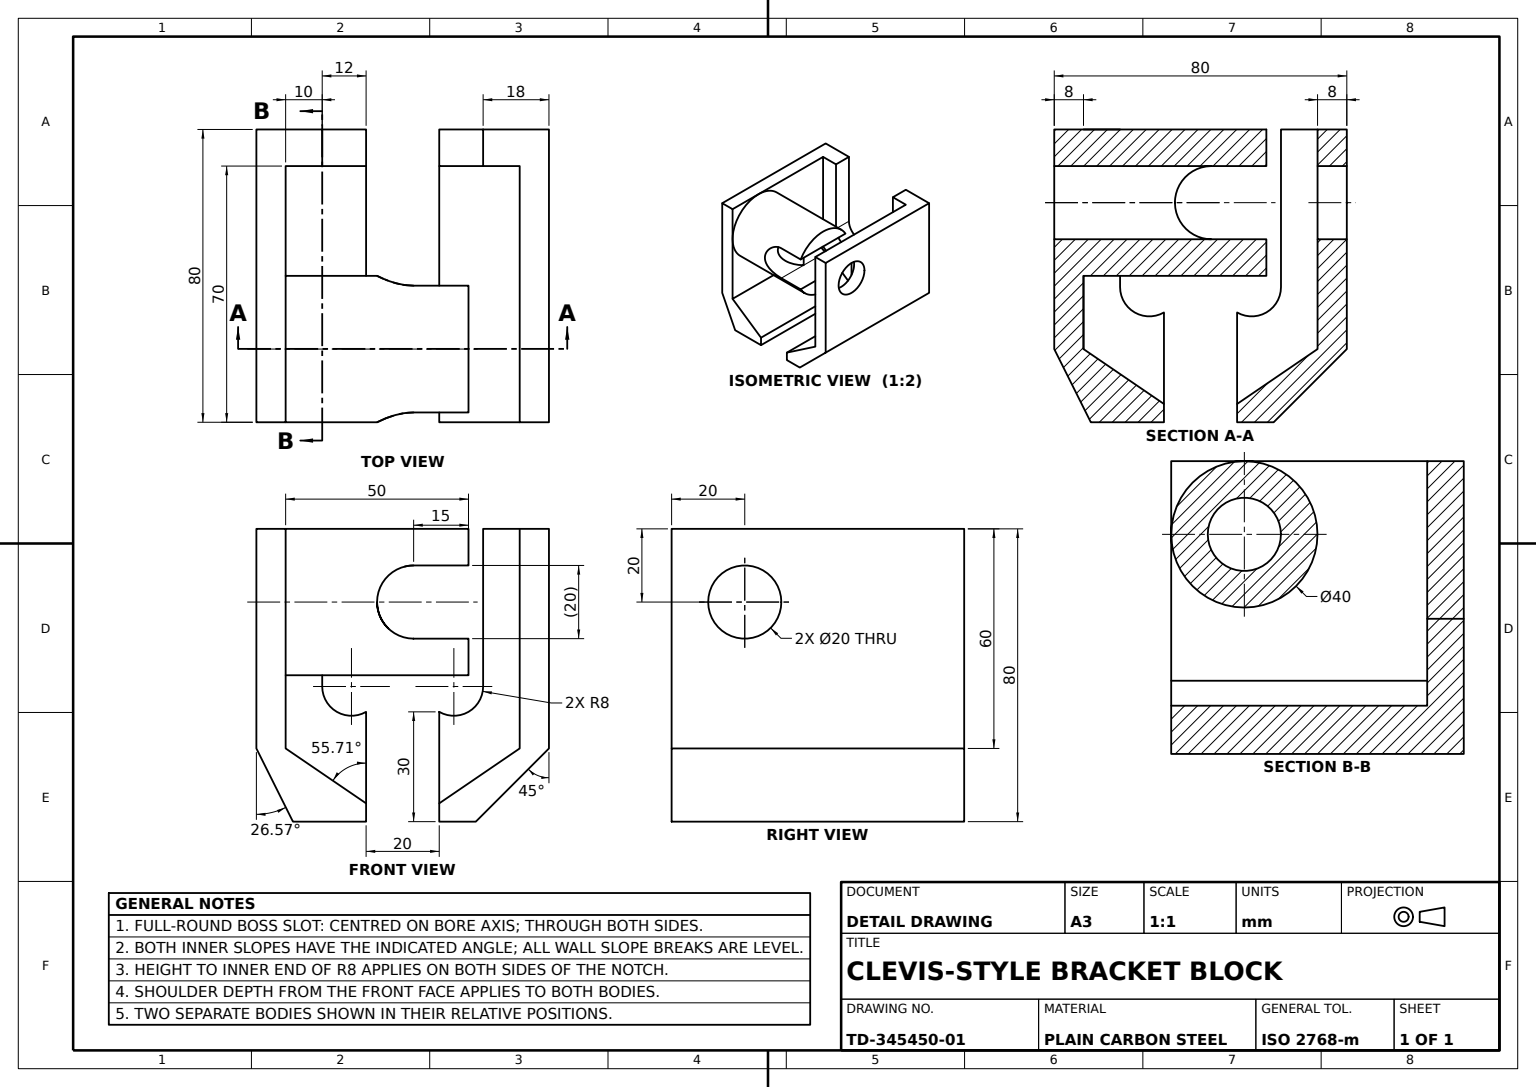
ISO-10303-21;
HEADER;
FILE_DESCRIPTION((''),'2;1');
FILE_NAME('','',(''),(''),'','','');
FILE_SCHEMA(('AUTOMOTIVE_DESIGN'));
ENDSEC;
DATA;
#1=APPLICATION_CONTEXT('');
#2=PRODUCT_CONTEXT('',#1,'mechanical');
#3=PRODUCT('','','',(#2));
#4=PRODUCT_DEFINITION_FORMATION('','',#3);
#5=PRODUCT_DEFINITION_CONTEXT('',#1,'design');
#6=PRODUCT_DEFINITION('','',#4,#5);
#7=PRODUCT_DEFINITION_SHAPE('','',#6);
#8=(LENGTH_UNIT()NAMED_UNIT(*)SI_UNIT(.MILLI.,.METRE.));
#9=(NAMED_UNIT(*)PLANE_ANGLE_UNIT()SI_UNIT($,.RADIAN.));
#10=(NAMED_UNIT(*)SI_UNIT($,.STERADIAN.)SOLID_ANGLE_UNIT());
#11=UNCERTAINTY_MEASURE_WITH_UNIT(LENGTH_MEASURE(1.E-05),#8,'distance_accuracy_value','');
#12=(GEOMETRIC_REPRESENTATION_CONTEXT(3)GLOBAL_UNCERTAINTY_ASSIGNED_CONTEXT((#11))GLOBAL_UNIT_ASSIGNED_CONTEXT((#8,#9,#10))REPRESENTATION_CONTEXT('',''));
#13=CARTESIAN_POINT('',(-40.,20.,42.));
#14=VERTEX_POINT('',#13);
#15=CARTESIAN_POINT('',(-40.,80.,42.));
#16=VERTEX_POINT('',#15);
#17=DIRECTION('',(0.,1.,0.));
#18=VECTOR('',#17,1000.);
#19=LINE('',#13,#18);
#20=EDGE_CURVE('',#14,#16,#19,.T.);
#21=ORIENTED_EDGE('',*,*,#20,.F.);
#22=CARTESIAN_POINT('',(-40.,5.,20.));
#23=VERTEX_POINT('',#22);
#24=DIRECTION('',(0.,0.563336825,0.826227343));
#25=VECTOR('',#24,1000.);
#26=LINE('',#22,#25);
#27=EDGE_CURVE('',#23,#14,#26,.T.);
#28=ORIENTED_EDGE('',*,*,#27,.F.);
#29=CARTESIAN_POINT('',(-40.,0.,20.));
#30=VERTEX_POINT('',#29);
#31=LINE('',#29,#18);
#32=EDGE_CURVE('',#30,#23,#31,.T.);
#33=ORIENTED_EDGE('',*,*,#32,.F.);
#34=CARTESIAN_POINT('',(-40.,0.,30.));
#35=VERTEX_POINT('',#34);
#36=CARTESIAN_POINT('',(-40.,0.,0.));
#37=DIRECTION('',(0.,0.,1.));
#38=VECTOR('',#37,1000.);
#39=LINE('',#36,#38);
#40=EDGE_CURVE('',#30,#35,#39,.T.);
#41=ORIENTED_EDGE('',*,*,#40,.T.);
#42=CARTESIAN_POINT('',(-40.,20.,50.));
#43=VERTEX_POINT('',#42);
#44=CARTESIAN_POINT('',(-40.,-15.,15.));
#45=DIRECTION('',(0.,-0.707106781,-0.707106781));
#46=VECTOR('',#45,1000.);
#47=LINE('',#44,#46);
#48=EDGE_CURVE('',#43,#35,#47,.T.);
#49=ORIENTED_EDGE('',*,*,#48,.F.);
#50=CARTESIAN_POINT('',(-40.,80.,50.));
#51=VERTEX_POINT('',#50);
#52=CARTESIAN_POINT('',(-40.,0.,50.));
#53=LINE('',#52,#18);
#54=EDGE_CURVE('',#43,#51,#53,.T.);
#55=ORIENTED_EDGE('',*,*,#54,.T.);
#56=CARTESIAN_POINT('',(-40.,80.,0.));
#57=DIRECTION('',(0.,0.,-1.));
#58=VECTOR('',#57,1000.);
#59=LINE('',#56,#58);
#60=EDGE_CURVE('',#51,#16,#59,.T.);
#61=ORIENTED_EDGE('',*,*,#60,.T.);
#62=EDGE_LOOP('',(#21,#28,#33,#41,#49,#55,#61));
#63=FACE_OUTER_BOUND('',#62,.T.);
#64=DIRECTION('',(1.,0.,0.));
#65=AXIS2_PLACEMENT_3D('',#36,#64,#57);
#66=PLANE('',#65);
#67=ADVANCED_FACE('',(#63),#66,.F.);
#68=CARTESIAN_POINT('',(-10.,60.,50.));
#69=VERTEX_POINT('',#68);
#70=CARTESIAN_POINT('',(-30.,60.,50.));
#71=VERTEX_POINT('',#70);
#72=CARTESIAN_POINT('',(-20.,60.,50.));
#73=DIRECTION('',(-1.,0.,0.));
#74=AXIS2_PLACEMENT_3D('',#72,#57,#73);
#75=CIRCLE('',#74,10.);
#76=EDGE_CURVE('',#69,#71,#75,.T.);
#77=ORIENTED_EDGE('',*,*,#76,.F.);
#78=CARTESIAN_POINT('',(-10.,60.,42.));
#79=VERTEX_POINT('',#78);
#80=CARTESIAN_POINT('',(-10.,60.,58.));
#81=LINE('',#80,#58);
#82=EDGE_CURVE('',#69,#79,#81,.T.);
#83=ORIENTED_EDGE('',*,*,#82,.T.);
#84=CARTESIAN_POINT('',(-30.,60.,42.));
#85=VERTEX_POINT('',#84);
#86=CARTESIAN_POINT('',(-20.,60.,42.));
#87=AXIS2_PLACEMENT_3D('',#86,#37,#64);
#88=CIRCLE('',#87,10.);
#89=EDGE_CURVE('',#85,#79,#88,.T.);
#90=ORIENTED_EDGE('',*,*,#89,.F.);
#91=CARTESIAN_POINT('',(-30.,60.,58.));
#92=LINE('',#91,#58);
#93=EDGE_CURVE('',#71,#85,#92,.T.);
#94=ORIENTED_EDGE('',*,*,#93,.F.);
#95=EDGE_LOOP('',(#77,#83,#90,#94));
#96=FACE_OUTER_BOUND('',#95,.T.);
#97=CARTESIAN_POINT('',(-20.,60.,58.));
#98=AXIS2_PLACEMENT_3D('',#97,#57,#73);
#99=CYLINDRICAL_SURFACE('',#98,10.);
#100=ADVANCED_FACE('',(#96),#99,.F.);
#101=CARTESIAN_POINT('',(30.,80.,42.));
#102=VERTEX_POINT('',#101);
#103=CARTESIAN_POINT('',(30.,80.,32.));
#104=VERTEX_POINT('',#103);
#105=CARTESIAN_POINT('',(30.,80.,12.853653));
#106=LINE('',#105,#58);
#107=EDGE_CURVE('',#102,#104,#106,.T.);
#108=ORIENTED_EDGE('',*,*,#107,.T.);
#109=CARTESIAN_POINT('',(30.,36.928203,32.));
#110=VERTEX_POINT('',#109);
#111=CARTESIAN_POINT('',(30.,0.,32.));
#112=LINE('',#111,#18);
#113=EDGE_CURVE('',#110,#104,#112,.T.);
#114=ORIENTED_EDGE('',*,*,#113,.F.);
#115=CARTESIAN_POINT('',(30.,30.,20.));
#116=VERTEX_POINT('',#115);
#117=CARTESIAN_POINT('',(30.,36.928203,24.));
#118=AXIS2_PLACEMENT_3D('',#117,#73,#57);
#119=CIRCLE('',#118,8.);
#120=EDGE_CURVE('',#116,#110,#119,.T.);
#121=ORIENTED_EDGE('',*,*,#120,.F.);
#122=CARTESIAN_POINT('',(30.,5.,20.));
#123=VERTEX_POINT('',#122);
#124=CARTESIAN_POINT('',(30.,0.,20.));
#125=DIRECTION('',(0.,-1.,0.));
#126=VECTOR('',#125,1000.);
#127=LINE('',#124,#126);
#128=EDGE_CURVE('',#116,#123,#127,.T.);
#129=ORIENTED_EDGE('',*,*,#128,.T.);
#130=CARTESIAN_POINT('',(30.,20.,42.));
#131=VERTEX_POINT('',#130);
#132=LINE('',#122,#25);
#133=EDGE_CURVE('',#123,#131,#132,.T.);
#134=ORIENTED_EDGE('',*,*,#133,.T.);
#135=LINE('',#130,#18);
#136=EDGE_CURVE('',#131,#102,#135,.T.);
#137=ORIENTED_EDGE('',*,*,#136,.T.);
#138=EDGE_LOOP('',(#108,#114,#121,#129,#134,#137));
#139=FACE_OUTER_BOUND('',#138,.T.);
#140=CARTESIAN_POINT('',(30.,20.,12.853653));
#141=AXIS2_PLACEMENT_3D('',#140,#64,#57);
#142=PLANE('',#141);
#143=ADVANCED_FACE('',(#139),#142,.F.);
#144=ORIENTED_EDGE('',*,*,#82,.F.);
#145=EDGE_CURVE('',#71,#69,#75,.T.);
#146=ORIENTED_EDGE('',*,*,#145,.F.);
#147=ORIENTED_EDGE('',*,*,#93,.T.);
#148=EDGE_CURVE('',#79,#85,#88,.T.);
#149=ORIENTED_EDGE('',*,*,#148,.F.);
#150=EDGE_LOOP('',(#144,#146,#147,#149));
#151=FACE_OUTER_BOUND('',#150,.T.);
#152=ADVANCED_FACE('',(#151),#99,.F.);
#153=ORIENTED_EDGE('',*,*,#89,.T.);
#154=ORIENTED_EDGE('',*,*,#148,.T.);
#155=EDGE_LOOP('',(#153,#154));
#156=FACE_BOUND('',#155,.T.);
#157=VECTOR('',#64,1000.);
#158=LINE('',#13,#157);
#159=EDGE_CURVE('',#14,#131,#158,.T.);
#160=ORIENTED_EDGE('',*,*,#159,.F.);
#161=ORIENTED_EDGE('',*,*,#20,.T.);
#162=LINE('',#15,#157);
#163=EDGE_CURVE('',#16,#102,#162,.T.);
#164=ORIENTED_EDGE('',*,*,#163,.T.);
#165=ORIENTED_EDGE('',*,*,#136,.F.);
#166=EDGE_LOOP('',(#160,#161,#164,#165));
#167=FACE_OUTER_BOUND('',#166,.T.);
#168=AXIS2_PLACEMENT_3D('',#13,#37,#64);
#169=PLANE('',#168);
#170=ADVANCED_FACE('',(#156,#167),#169,.F.);
#171=CARTESIAN_POINT('',(40.,0.,30.));
#172=VERTEX_POINT('',#171);
#173=LINE('',#34,#157);
#174=EDGE_CURVE('',#35,#172,#173,.T.);
#175=ORIENTED_EDGE('',*,*,#174,.F.);
#176=ORIENTED_EDGE('',*,*,#40,.F.);
#177=CARTESIAN_POINT('',(40.,0.,20.));
#178=VERTEX_POINT('',#177);
#179=LINE('',#29,#157);
#180=EDGE_CURVE('',#30,#178,#179,.T.);
#181=ORIENTED_EDGE('',*,*,#180,.T.);
#182=CARTESIAN_POINT('',(40.,0.,0.));
#183=LINE('',#182,#38);
#184=EDGE_CURVE('',#178,#172,#183,.T.);
#185=ORIENTED_EDGE('',*,*,#184,.T.);
#186=EDGE_LOOP('',(#175,#176,#181,#185));
#187=FACE_OUTER_BOUND('',#186,.T.);
#188=AXIS2_PLACEMENT_3D('',#36,#17,#37);
#189=PLANE('',#188);
#190=ADVANCED_FACE('',(#187),#189,.F.);
#191=ORIENTED_EDGE('',*,*,#76,.T.);
#192=ORIENTED_EDGE('',*,*,#145,.T.);
#193=EDGE_LOOP('',(#191,#192));
#194=FACE_BOUND('',#193,.T.);
#195=CARTESIAN_POINT('',(40.,80.,50.));
#196=VERTEX_POINT('',#195);
#197=LINE('',#50,#157);
#198=EDGE_CURVE('',#51,#196,#197,.T.);
#199=ORIENTED_EDGE('',*,*,#198,.F.);
#200=ORIENTED_EDGE('',*,*,#54,.F.);
#201=CARTESIAN_POINT('',(40.,20.,50.));
#202=VERTEX_POINT('',#201);
#203=LINE('',#42,#157);
#204=EDGE_CURVE('',#43,#202,#203,.T.);
#205=ORIENTED_EDGE('',*,*,#204,.T.);
#206=CARTESIAN_POINT('',(40.,0.,50.));
#207=LINE('',#206,#18);
#208=EDGE_CURVE('',#202,#196,#207,.T.);
#209=ORIENTED_EDGE('',*,*,#208,.T.);
#210=EDGE_LOOP('',(#199,#200,#205,#209));
#211=FACE_OUTER_BOUND('',#210,.T.);
#212=AXIS2_PLACEMENT_3D('',#52,#57,#73);
#213=PLANE('',#212);
#214=ADVANCED_FACE('',(#194,#211),#213,.F.);
#215=ORIENTED_EDGE('',*,*,#32,.T.);
#216=VECTOR('',#73,1000.);
#217=LINE('',#122,#216);
#218=EDGE_CURVE('',#123,#23,#217,.T.);
#219=ORIENTED_EDGE('',*,*,#218,.F.);
#220=ORIENTED_EDGE('',*,*,#128,.F.);
#221=CARTESIAN_POINT('',(40.,30.,20.));
#222=VERTEX_POINT('',#221);
#223=CARTESIAN_POINT('',(-40.,30.,20.));
#224=LINE('',#223,#157);
#225=EDGE_CURVE('',#116,#222,#224,.T.);
#226=ORIENTED_EDGE('',*,*,#225,.T.);
#227=LINE('',#177,#18);
#228=EDGE_CURVE('',#178,#222,#227,.T.);
#229=ORIENTED_EDGE('',*,*,#228,.F.);
#230=ORIENTED_EDGE('',*,*,#180,.F.);
#231=EDGE_LOOP('',(#215,#219,#220,#226,#229,#230));
#232=FACE_OUTER_BOUND('',#231,.T.);
#233=AXIS2_PLACEMENT_3D('',#29,#57,#73);
#234=PLANE('',#233);
#235=ADVANCED_FACE('',(#232),#234,.T.);
#236=ORIENTED_EDGE('',*,*,#133,.F.);
#237=ORIENTED_EDGE('',*,*,#218,.T.);
#238=ORIENTED_EDGE('',*,*,#27,.T.);
#239=ORIENTED_EDGE('',*,*,#159,.T.);
#240=EDGE_LOOP('',(#236,#237,#238,#239));
#241=FACE_OUTER_BOUND('',#240,.T.);
#242=DIRECTION('',(0.,-0.826227343,0.563336825));
#243=DIRECTION('',(0.,-0.563336825,-0.826227343));
#244=AXIS2_PLACEMENT_3D('',#122,#242,#243);
#245=PLANE('',#244);
#246=ADVANCED_FACE('',(#241),#245,.F.);
#247=ORIENTED_EDGE('',*,*,#60,.F.);
#248=ORIENTED_EDGE('',*,*,#198,.T.);
#249=CARTESIAN_POINT('',(40.,80.,32.));
#250=VERTEX_POINT('',#249);
#251=CARTESIAN_POINT('',(40.,80.,0.));
#252=LINE('',#251,#58);
#253=EDGE_CURVE('',#196,#250,#252,.T.);
#254=ORIENTED_EDGE('',*,*,#253,.T.);
#255=CARTESIAN_POINT('',(-40.,80.,32.));
#256=LINE('',#255,#157);
#257=EDGE_CURVE('',#104,#250,#256,.T.);
#258=ORIENTED_EDGE('',*,*,#257,.F.);
#259=ORIENTED_EDGE('',*,*,#107,.F.);
#260=ORIENTED_EDGE('',*,*,#163,.F.);
#261=EDGE_LOOP('',(#247,#248,#254,#258,#259,#260));
#262=FACE_OUTER_BOUND('',#261,.T.);
#263=AXIS2_PLACEMENT_3D('',#56,#125,#57);
#264=PLANE('',#263);
#265=ADVANCED_FACE('',(#262),#264,.F.);
#266=ORIENTED_EDGE('',*,*,#204,.F.);
#267=ORIENTED_EDGE('',*,*,#48,.T.);
#268=ORIENTED_EDGE('',*,*,#174,.T.);
#269=CARTESIAN_POINT('',(40.,-15.,15.));
#270=LINE('',#269,#46);
#271=EDGE_CURVE('',#202,#172,#270,.T.);
#272=ORIENTED_EDGE('',*,*,#271,.F.);
#273=EDGE_LOOP('',(#266,#267,#268,#272));
#274=FACE_OUTER_BOUND('',#273,.T.);
#275=DIRECTION('',(0.,-0.707106781,0.707106781));
#276=AXIS2_PLACEMENT_3D('',#44,#275,#45);
#277=PLANE('',#276);
#278=ADVANCED_FACE('',(#274),#277,.T.);
#279=ORIENTED_EDGE('',*,*,#228,.T.);
#280=CARTESIAN_POINT('',(40.,36.928203,32.));
#281=VERTEX_POINT('',#280);
#282=CARTESIAN_POINT('',(40.,36.928203,24.));
#283=AXIS2_PLACEMENT_3D('',#282,#64,#57);
#284=CIRCLE('',#283,8.);
#285=EDGE_CURVE('',#281,#222,#284,.T.);
#286=ORIENTED_EDGE('',*,*,#285,.F.);
#287=CARTESIAN_POINT('',(40.,0.,32.));
#288=LINE('',#287,#126);
#289=EDGE_CURVE('',#250,#281,#288,.T.);
#290=ORIENTED_EDGE('',*,*,#289,.F.);
#291=ORIENTED_EDGE('',*,*,#253,.F.);
#292=ORIENTED_EDGE('',*,*,#208,.F.);
#293=ORIENTED_EDGE('',*,*,#271,.T.);
#294=ORIENTED_EDGE('',*,*,#184,.F.);
#295=EDGE_LOOP('',(#279,#286,#290,#291,#292,#293,#294));
#296=FACE_OUTER_BOUND('',#295,.T.);
#297=AXIS2_PLACEMENT_3D('',#182,#64,#57);
#298=PLANE('',#297);
#299=ADVANCED_FACE('',(#296),#298,.T.);
#300=ORIENTED_EDGE('',*,*,#113,.T.);
#301=ORIENTED_EDGE('',*,*,#257,.T.);
#302=ORIENTED_EDGE('',*,*,#289,.T.);
#303=CARTESIAN_POINT('',(-40.,36.928203,32.));
#304=LINE('',#303,#157);
#305=EDGE_CURVE('',#110,#281,#304,.T.);
#306=ORIENTED_EDGE('',*,*,#305,.F.);
#307=EDGE_LOOP('',(#300,#301,#302,#306));
#308=FACE_OUTER_BOUND('',#307,.T.);
#309=CARTESIAN_POINT('',(-40.,0.,32.));
#310=AXIS2_PLACEMENT_3D('',#309,#37,#64);
#311=PLANE('',#310);
#312=ADVANCED_FACE('',(#308),#311,.F.);
#313=ORIENTED_EDGE('',*,*,#285,.T.);
#314=ORIENTED_EDGE('',*,*,#225,.F.);
#315=ORIENTED_EDGE('',*,*,#120,.T.);
#316=ORIENTED_EDGE('',*,*,#305,.T.);
#317=EDGE_LOOP('',(#313,#314,#315,#316));
#318=FACE_OUTER_BOUND('',#317,.T.);
#319=CARTESIAN_POINT('',(-40.,36.928203,24.));
#320=AXIS2_PLACEMENT_3D('',#319,#64,#57);
#321=CYLINDRICAL_SURFACE('',#320,8.);
#322=ADVANCED_FACE('',(#318),#321,.F.);
#323=CLOSED_SHELL('',(#67,#100,#143,#152,#170,#190,#214,#235,#246,#265,#278,#299,#312,#322));
#324=MANIFOLD_SOLID_BREP('',#323);
#325=CARTESIAN_POINT('',(-2.679492,70.,13.));
#326=VERTEX_POINT('',#325);
#327=CARTESIAN_POINT('',(0.,60.,3.));
#328=VERTEX_POINT('',#327);
#329=CARTESIAN_POINT('',(-2.679492,70.,12.326451));
#330=CARTESIAN_POINT('',(-2.64015,69.932676,11.666936));
#331=CARTESIAN_POINT('',(-2.530016,69.736799,10.697061));
#332=CARTESIAN_POINT('',(-2.484794,69.655561,10.377023));
#333=CARTESIAN_POINT('',(-2.378767,69.460679,9.743406));
#334=CARTESIAN_POINT('',(-2.318419,69.347832,9.432838));
#335=CARTESIAN_POINT('',(-2.121545,68.96894,8.529595));
#336=CARTESIAN_POINT('',(-1.968469,68.661548,7.960234));
#337=CARTESIAN_POINT('',(-1.72064,68.118167,7.151857));
#338=CARTESIAN_POINT('',(-1.635194,67.923582,6.890945));
#339=CARTESIAN_POINT('',(-1.463889,67.51411,6.393802));
#340=CARTESIAN_POINT('',(-1.377643,67.298395,6.156297));
#341=CARTESIAN_POINT('',(-1.206215,66.844882,5.70271));
#342=CARTESIAN_POINT('',(-1.121029,66.607085,5.48663));
#343=CARTESIAN_POINT('',(-0.953869,66.108522,5.075969));
#344=CARTESIAN_POINT('',(-0.871478,65.846241,4.880453));
#345=CARTESIAN_POINT('',(-0.636562,65.037136,4.336887));
#346=CARTESIAN_POINT('',(-0.495718,64.467502,4.029686));
#347=CARTESIAN_POINT('',(-0.318011,63.565556,3.651573));
#348=CARTESIAN_POINT('',(-0.264369,63.256938,3.539427));
#349=CARTESIAN_POINT('',(-0.170113,62.622666,3.344343));
#350=CARTESIAN_POINT('',(-0.129818,62.298314,3.262065));
#351=CARTESIAN_POINT('',(-0.033251,61.324568,3.066017));
#352=CARTESIAN_POINT('',(0.,60.666743,3.));
#353=B_SPLINE_CURVE_WITH_KNOTS('',3,(#325,#329,#330,#331,#332,#333,#334,#335,#336,#337,#338,#339,#340,#341,#342,#343,#344,#345,#346,#347,#348,#349,#350,#351,#352,#327),.UNSPECIFIED.,.F.,.F.,(4,2,2,2,2,2,2,2,2,2,2,2,4),(0.,0.001988686,0.00298303,0.003977373,0.005966059,0.006960402,0.007954745,0.008949089,0.009943432,0.011932118,0.012926461,0.013920805,0.015909491),.UNSPECIFIED.);
#354=EDGE_CURVE('',#326,#328,#353,.T.);
#355=ORIENTED_EDGE('',*,*,#354,.T.);
#356=CARTESIAN_POINT('',(0.,60.,-22.));
#357=VERTEX_POINT('',#356);
#358=CARTESIAN_POINT('',(0.,60.,28.));
#359=LINE('',#358,#58);
#360=EDGE_CURVE('',#328,#357,#359,.T.);
#361=ORIENTED_EDGE('',*,*,#360,.T.);
#362=CARTESIAN_POINT('',(-20.,80.,-22.));
#363=VERTEX_POINT('',#362);
#364=CARTESIAN_POINT('',(-20.,60.,-22.));
#365=AXIS2_PLACEMENT_3D('',#364,#37,#73);
#366=CIRCLE('',#365,20.);
#367=EDGE_CURVE('',#357,#363,#366,.T.);
#368=ORIENTED_EDGE('',*,*,#367,.T.);
#369=CARTESIAN_POINT('',(-40.,60.,-22.));
#370=VERTEX_POINT('',#369);
#371=AXIS2_PLACEMENT_3D('',#364,#37,#64);
#372=CIRCLE('',#371,20.);
#373=EDGE_CURVE('',#363,#370,#372,.T.);
#374=ORIENTED_EDGE('',*,*,#373,.T.);
#375=CARTESIAN_POINT('',(-40.,60.,3.));
#376=VERTEX_POINT('',#375);
#377=CARTESIAN_POINT('',(-40.,60.,28.));
#378=LINE('',#377,#58);
#379=EDGE_CURVE('',#376,#370,#378,.T.);
#380=ORIENTED_EDGE('',*,*,#379,.F.);
#381=CARTESIAN_POINT('',(-37.320508,70.,13.));
#382=VERTEX_POINT('',#381);
#383=CARTESIAN_POINT('',(-40.,60.332731,3.));
#384=CARTESIAN_POINT('',(-39.991541,60.669812,3.016886));
#385=CARTESIAN_POINT('',(-39.958266,61.333415,3.08369));
#386=CARTESIAN_POINT('',(-39.933565,61.660889,3.133376));
#387=CARTESIAN_POINT('',(-39.869095,62.307518,3.264283));
#388=CARTESIAN_POINT('',(-39.829323,62.626671,3.345506));
#389=CARTESIAN_POINT('',(-39.735627,63.256761,3.539442));
#390=CARTESIAN_POINT('',(-39.681337,63.569376,3.652932));
#391=CARTESIAN_POINT('',(-39.501841,64.478854,4.034937));
#392=CARTESIAN_POINT('',(-39.360277,65.048984,4.343981));
#393=CARTESIAN_POINT('',(-39.126053,65.85425,4.886278));
#394=CARTESIAN_POINT('',(-39.043918,66.115438,5.081272));
#395=CARTESIAN_POINT('',(-38.876246,66.614887,5.493463));
#396=CARTESIAN_POINT('',(-38.790952,66.852641,5.710006));
#397=CARTESIAN_POINT('',(-38.533965,67.531694,6.390584));
#398=CARTESIAN_POINT('',(-38.361043,67.939173,6.885171));
#399=CARTESIAN_POINT('',(-38.11329,68.482235,7.693675));
#400=CARTESIAN_POINT('',(-38.033379,68.650225,7.97227));
#401=CARTESIAN_POINT('',(-37.883077,68.956825,8.54133));
#402=CARTESIAN_POINT('',(-37.812381,69.096099,8.832768));
#403=CARTESIAN_POINT('',(-37.682206,69.346632,9.429941));
#404=CARTESIAN_POINT('',(-37.622724,69.457893,9.735675));
#405=CARTESIAN_POINT('',(-37.517466,69.651451,10.362379));
#406=CARTESIAN_POINT('',(-37.471499,69.734089,10.685153));
#407=CARTESIAN_POINT('',(-37.359786,69.93282,11.664684));
#408=CARTESIAN_POINT('',(-37.320508,70.,12.327306));
#409=B_SPLINE_CURVE_WITH_KNOTS('',3,(#375,#383,#384,#385,#386,#387,#388,#389,#390,#391,#392,#393,#394,#395,#396,#397,#398,#399,#400,#401,#402,#403,#404,#405,#406,#407,#408,#381),.UNSPECIFIED.,.F.,.F.,(4,2,2,2,2,2,2,2,2,2,2,2,2,4),(0.015909491,0.016901923,0.017894356,0.018886788,0.019879221,0.021864085,0.022856518,0.02384895,0.025833815,0.026826248,0.02781868,0.028811112,0.029803545,0.03178841),.UNSPECIFIED.);
#410=EDGE_CURVE('',#376,#382,#409,.T.);
#411=ORIENTED_EDGE('',*,*,#410,.T.);
#412=CARTESIAN_POINT('',(-37.320508,70.,28.));
#413=VERTEX_POINT('',#412);
#414=LINE('',#412,#38);
#415=EDGE_CURVE('',#382,#413,#414,.T.);
#416=ORIENTED_EDGE('',*,*,#415,.T.);
#417=CARTESIAN_POINT('',(-2.679492,70.,28.));
#418=VERTEX_POINT('',#417);
#419=CARTESIAN_POINT('',(-20.,60.,28.));
#420=AXIS2_PLACEMENT_3D('',#419,#37,#64);
#421=CIRCLE('',#420,20.);
#422=EDGE_CURVE('',#418,#413,#421,.T.);
#423=ORIENTED_EDGE('',*,*,#422,.F.);
#424=LINE('',#417,#58);
#425=EDGE_CURVE('',#418,#326,#424,.T.);
#426=ORIENTED_EDGE('',*,*,#425,.T.);
#427=EDGE_LOOP('',(#355,#361,#368,#374,#380,#411,#416,#423,#426));
#428=FACE_OUTER_BOUND('',#427,.T.);
#429=AXIS2_PLACEMENT_3D('',#419,#57,#73);
#430=CYLINDRICAL_SURFACE('',#429,20.);
#431=ADVANCED_FACE('',(#428),#430,.T.);
#432=VERTEX_POINT('',#36);
#433=CARTESIAN_POINT('',(-40.,0.,-20.));
#434=VERTEX_POINT('',#433);
#435=LINE('',#36,#58);
#436=EDGE_CURVE('',#432,#434,#435,.T.);
#437=ORIENTED_EDGE('',*,*,#436,.F.);
#438=CARTESIAN_POINT('',(-40.,5.,0.));
#439=VERTEX_POINT('',#438);
#440=LINE('',#36,#126);
#441=EDGE_CURVE('',#439,#432,#440,.T.);
#442=ORIENTED_EDGE('',*,*,#441,.F.);
#443=CARTESIAN_POINT('',(-40.,20.,-22.));
#444=VERTEX_POINT('',#443);
#445=CARTESIAN_POINT('',(-40.,3.413258,2.327221));
#446=DIRECTION('',(0.,0.563336825,-0.826227343));
#447=VECTOR('',#446,1000.);
#448=LINE('',#445,#447);
#449=EDGE_CURVE('',#439,#444,#448,.T.);
#450=ORIENTED_EDGE('',*,*,#449,.T.);
#451=LINE('',#443,#18);
#452=EDGE_CURVE('',#444,#370,#451,.T.);
#453=ORIENTED_EDGE('',*,*,#452,.T.);
#454=CARTESIAN_POINT('',(-40.,80.,-22.));
#455=VERTEX_POINT('',#454);
#456=EDGE_CURVE('',#370,#455,#451,.T.);
#457=ORIENTED_EDGE('',*,*,#456,.T.);
#458=CARTESIAN_POINT('',(-40.,80.,-30.));
#459=VERTEX_POINT('',#458);
#460=LINE('',#458,#38);
#461=EDGE_CURVE('',#459,#455,#460,.T.);
#462=ORIENTED_EDGE('',*,*,#461,.F.);
#463=CARTESIAN_POINT('',(-40.,20.,-30.));
#464=VERTEX_POINT('',#463);
#465=LINE('',#463,#18);
#466=EDGE_CURVE('',#464,#459,#465,.T.);
#467=ORIENTED_EDGE('',*,*,#466,.F.);
#468=DIRECTION('',(0.,0.894427191,-0.447213595));
#469=VECTOR('',#468,1000.);
#470=LINE('',#463,#469);
#471=EDGE_CURVE('',#434,#464,#470,.T.);
#472=ORIENTED_EDGE('',*,*,#471,.F.);
#473=EDGE_LOOP('',(#437,#442,#450,#453,#457,#462,#467,#472));
#474=FACE_OUTER_BOUND('',#473,.T.);
#475=CARTESIAN_POINT('',(-40.,36.928203,-4.));
#476=AXIS2_PLACEMENT_3D('',#475,#64,#57);
#477=PLANE('',#476);
#478=ADVANCED_FACE('',(#474),#477,.F.);
#479=VERTEX_POINT('',#182);
#480=CARTESIAN_POINT('',(40.,0.,-20.));
#481=VERTEX_POINT('',#480);
#482=LINE('',#182,#58);
#483=EDGE_CURVE('',#479,#481,#482,.T.);
#484=ORIENTED_EDGE('',*,*,#483,.T.);
#485=CARTESIAN_POINT('',(40.,20.,-30.));
#486=VERTEX_POINT('',#485);
#487=LINE('',#485,#469);
#488=EDGE_CURVE('',#481,#486,#487,.T.);
#489=ORIENTED_EDGE('',*,*,#488,.T.);
#490=CARTESIAN_POINT('',(40.,80.,-30.));
#491=VERTEX_POINT('',#490);
#492=LINE('',#485,#18);
#493=EDGE_CURVE('',#486,#491,#492,.T.);
#494=ORIENTED_EDGE('',*,*,#493,.T.);
#495=CARTESIAN_POINT('',(40.,80.,-12.));
#496=VERTEX_POINT('',#495);
#497=LINE('',#490,#38);
#498=EDGE_CURVE('',#491,#496,#497,.T.);
#499=ORIENTED_EDGE('',*,*,#498,.T.);
#500=CARTESIAN_POINT('',(40.,36.928203,-12.));
#501=VERTEX_POINT('',#500);
#502=LINE('',#495,#126);
#503=EDGE_CURVE('',#496,#501,#502,.T.);
#504=ORIENTED_EDGE('',*,*,#503,.T.);
#505=CARTESIAN_POINT('',(40.,30.,0.));
#506=VERTEX_POINT('',#505);
#507=CARTESIAN_POINT('',(40.,36.928203,-4.));
#508=AXIS2_PLACEMENT_3D('',#507,#73,#57);
#509=CIRCLE('',#508,8.);
#510=EDGE_CURVE('',#501,#506,#509,.T.);
#511=ORIENTED_EDGE('',*,*,#510,.T.);
#512=LINE('',#182,#126);
#513=EDGE_CURVE('',#506,#479,#512,.T.);
#514=ORIENTED_EDGE('',*,*,#513,.T.);
#515=EDGE_LOOP('',(#484,#489,#494,#499,#504,#511,#514));
#516=FACE_OUTER_BOUND('',#515,.T.);
#517=AXIS2_PLACEMENT_3D('',#507,#64,#57);
#518=PLANE('',#517);
#519=ADVANCED_FACE('',(#516),#518,.T.);
#520=CARTESIAN_POINT('',(-10.,60.,3.));
#521=VERTEX_POINT('',#520);
#522=CARTESIAN_POINT('',(-10.,60.,-30.));
#523=VERTEX_POINT('',#522);
#524=EDGE_CURVE('',#521,#523,#81,.T.);
#525=ORIENTED_EDGE('',*,*,#524,.F.);
#526=CARTESIAN_POINT('',(-20.,70.,13.));
#527=VERTEX_POINT('',#526);
#528=CARTESIAN_POINT('',(-14.142136,70.,7.142136));
#529=CARTESIAN_POINT('',(-10.,65.857864,3.));
#530=(BOUNDED_CURVE()B_SPLINE_CURVE(3,(#526,#528,#529,#520),.UNSPECIFIED.,.F.,.T.)B_SPLINE_CURVE_WITH_KNOTS((4,4),(4.71238898,6.283185307),.UNSPECIFIED.)CURVE()GEOMETRIC_REPRESENTATION_ITEM()RATIONAL_B_SPLINE_CURVE((1.,0.804737854,0.804737854,1.))REPRESENTATION_ITEM(''));
#531=EDGE_CURVE('',#527,#521,#530,.T.);
#532=ORIENTED_EDGE('',*,*,#531,.F.);
#533=CARTESIAN_POINT('',(-30.,60.,3.));
#534=VERTEX_POINT('',#533);
#535=CARTESIAN_POINT('',(-30.,65.857864,3.));
#536=CARTESIAN_POINT('',(-25.857864,70.,7.142136));
#537=(BOUNDED_CURVE()B_SPLINE_CURVE(3,(#533,#535,#536,#526),.UNSPECIFIED.,.F.,.T.)B_SPLINE_CURVE_WITH_KNOTS((4,4),(3.141592654,4.71238898),.UNSPECIFIED.)CURVE()GEOMETRIC_REPRESENTATION_ITEM()RATIONAL_B_SPLINE_CURVE((1.,0.804737854,0.804737854,1.))REPRESENTATION_ITEM(''));
#538=EDGE_CURVE('',#534,#527,#537,.T.);
#539=ORIENTED_EDGE('',*,*,#538,.F.);
#540=CARTESIAN_POINT('',(-30.,60.,-30.));
#541=VERTEX_POINT('',#540);
#542=EDGE_CURVE('',#534,#541,#92,.T.);
#543=ORIENTED_EDGE('',*,*,#542,.T.);
#544=CARTESIAN_POINT('',(-20.,60.,-30.));
#545=AXIS2_PLACEMENT_3D('',#544,#57,#73);
#546=CIRCLE('',#545,10.);
#547=EDGE_CURVE('',#541,#523,#546,.T.);
#548=ORIENTED_EDGE('',*,*,#547,.T.);
#549=EDGE_LOOP('',(#525,#532,#539,#543,#548));
#550=FACE_OUTER_BOUND('',#549,.T.);
#551=ADVANCED_FACE('',(#550),#99,.F.);
#552=CARTESIAN_POINT('',(-37.320508,50.,13.));
#553=VERTEX_POINT('',#552);
#554=CARTESIAN_POINT('',(-37.320508,50.,12.326451));
#555=CARTESIAN_POINT('',(-37.35985,50.067324,11.666936));
#556=CARTESIAN_POINT('',(-37.469984,50.263201,10.697061));
#557=CARTESIAN_POINT('',(-37.515206,50.344439,10.377023));
#558=CARTESIAN_POINT('',(-37.621233,50.539321,9.743406));
#559=CARTESIAN_POINT('',(-37.681581,50.652168,9.432838));
#560=CARTESIAN_POINT('',(-37.878455,51.03106,8.529595));
#561=CARTESIAN_POINT('',(-38.031531,51.338452,7.960234));
#562=CARTESIAN_POINT('',(-38.27936,51.881833,7.151857));
#563=CARTESIAN_POINT('',(-38.364806,52.076418,6.890945));
#564=CARTESIAN_POINT('',(-38.536111,52.48589,6.393802));
#565=CARTESIAN_POINT('',(-38.622357,52.701605,6.156297));
#566=CARTESIAN_POINT('',(-38.793785,53.155118,5.70271));
#567=CARTESIAN_POINT('',(-38.878971,53.392915,5.48663));
#568=CARTESIAN_POINT('',(-39.046131,53.891478,5.075969));
#569=CARTESIAN_POINT('',(-39.128522,54.153759,4.880453));
#570=CARTESIAN_POINT('',(-39.363438,54.962864,4.336887));
#571=CARTESIAN_POINT('',(-39.504282,55.532498,4.029686));
#572=CARTESIAN_POINT('',(-39.681989,56.434444,3.651573));
#573=CARTESIAN_POINT('',(-39.735631,56.743062,3.539427));
#574=CARTESIAN_POINT('',(-39.829887,57.377334,3.344343));
#575=CARTESIAN_POINT('',(-39.870182,57.701686,3.262065));
#576=CARTESIAN_POINT('',(-39.966749,58.675432,3.066017));
#577=CARTESIAN_POINT('',(-40.,59.333257,3.));
#578=B_SPLINE_CURVE_WITH_KNOTS('',3,(#552,#554,#555,#556,#557,#558,#559,#560,#561,#562,#563,#564,#565,#566,#567,#568,#569,#570,#571,#572,#573,#574,#575,#576,#577,#375),.UNSPECIFIED.,.F.,.F.,(4,2,2,2,2,2,2,2,2,2,2,2,4),(0.,0.001988686,0.00298303,0.003977373,0.005966059,0.006960402,0.007954745,0.008949089,0.009943432,0.011932118,0.012926461,0.013920805,0.015909491),.UNSPECIFIED.);
#579=EDGE_CURVE('',#553,#376,#578,.T.);
#580=ORIENTED_EDGE('',*,*,#579,.T.);
#581=ORIENTED_EDGE('',*,*,#379,.T.);
#582=EDGE_CURVE('',#370,#357,#366,.T.);
#583=ORIENTED_EDGE('',*,*,#582,.T.);
#584=ORIENTED_EDGE('',*,*,#360,.F.);
#585=CARTESIAN_POINT('',(-2.679492,50.,13.));
#586=VERTEX_POINT('',#585);
#587=CARTESIAN_POINT('',(0.,59.667269,3.));
#588=CARTESIAN_POINT('',(-0.008459,59.330188,3.016886));
#589=CARTESIAN_POINT('',(-0.041734,58.666585,3.08369));
#590=CARTESIAN_POINT('',(-0.066435,58.339111,3.133376));
#591=CARTESIAN_POINT('',(-0.130905,57.692482,3.264283));
#592=CARTESIAN_POINT('',(-0.170677,57.373329,3.345506));
#593=CARTESIAN_POINT('',(-0.264373,56.743239,3.539442));
#594=CARTESIAN_POINT('',(-0.318663,56.430624,3.652932));
#595=CARTESIAN_POINT('',(-0.498159,55.521146,4.034937));
#596=CARTESIAN_POINT('',(-0.639723,54.951016,4.343981));
#597=CARTESIAN_POINT('',(-0.873947,54.14575,4.886278));
#598=CARTESIAN_POINT('',(-0.956082,53.884562,5.081272));
#599=CARTESIAN_POINT('',(-1.123754,53.385113,5.493463));
#600=CARTESIAN_POINT('',(-1.209048,53.147359,5.710006));
#601=CARTESIAN_POINT('',(-1.466035,52.468306,6.390584));
#602=CARTESIAN_POINT('',(-1.638957,52.060827,6.885171));
#603=CARTESIAN_POINT('',(-1.88671,51.517765,7.693675));
#604=CARTESIAN_POINT('',(-1.966621,51.349775,7.97227));
#605=CARTESIAN_POINT('',(-2.116923,51.043175,8.54133));
#606=CARTESIAN_POINT('',(-2.187619,50.903901,8.832768));
#607=CARTESIAN_POINT('',(-2.317794,50.653368,9.429941));
#608=CARTESIAN_POINT('',(-2.377276,50.542107,9.735675));
#609=CARTESIAN_POINT('',(-2.482534,50.348549,10.362379));
#610=CARTESIAN_POINT('',(-2.528501,50.265911,10.685153));
#611=CARTESIAN_POINT('',(-2.640214,50.06718,11.664684));
#612=CARTESIAN_POINT('',(-2.679492,50.,12.327306));
#613=B_SPLINE_CURVE_WITH_KNOTS('',3,(#327,#587,#588,#589,#590,#591,#592,#593,#594,#595,#596,#597,#598,#599,#600,#601,#602,#603,#604,#605,#606,#607,#608,#609,#610,#611,#612,#585),.UNSPECIFIED.,.F.,.F.,(4,2,2,2,2,2,2,2,2,2,2,2,2,4),(0.015909491,0.016901923,0.017894356,0.018886788,0.019879221,0.021864085,0.022856518,0.02384895,0.025833815,0.026826248,0.02781868,0.028811112,0.029803545,0.03178841),.UNSPECIFIED.);
#614=EDGE_CURVE('',#328,#586,#613,.T.);
#615=ORIENTED_EDGE('',*,*,#614,.T.);
#616=CARTESIAN_POINT('',(-2.679492,50.,28.));
#617=VERTEX_POINT('',#616);
#618=LINE('',#616,#38);
#619=EDGE_CURVE('',#586,#617,#618,.T.);
#620=ORIENTED_EDGE('',*,*,#619,.T.);
#621=CARTESIAN_POINT('',(-37.320508,50.,28.));
#622=VERTEX_POINT('',#621);
#623=EDGE_CURVE('',#622,#617,#421,.T.);
#624=ORIENTED_EDGE('',*,*,#623,.F.);
#625=LINE('',#621,#58);
#626=EDGE_CURVE('',#622,#553,#625,.T.);
#627=ORIENTED_EDGE('',*,*,#626,.T.);
#628=EDGE_LOOP('',(#580,#581,#583,#584,#615,#620,#624,#627));
#629=FACE_OUTER_BOUND('',#628,.T.);
#630=ADVANCED_FACE('',(#629),#430,.T.);
#631=CARTESIAN_POINT('',(-20.,50.,13.));
#632=VERTEX_POINT('',#631);
#633=CARTESIAN_POINT('',(-10.,54.142136,3.));
#634=CARTESIAN_POINT('',(-14.142136,50.,7.142136));
#635=(BOUNDED_CURVE()B_SPLINE_CURVE(3,(#520,#633,#634,#631),.UNSPECIFIED.,.F.,.T.)B_SPLINE_CURVE_WITH_KNOTS((4,4),(0.,1.570796327),.UNSPECIFIED.)CURVE()GEOMETRIC_REPRESENTATION_ITEM()RATIONAL_B_SPLINE_CURVE((1.,0.804737854,0.804737854,1.))REPRESENTATION_ITEM(''));
#636=EDGE_CURVE('',#521,#632,#635,.T.);
#637=ORIENTED_EDGE('',*,*,#636,.F.);
#638=ORIENTED_EDGE('',*,*,#524,.T.);
#639=EDGE_CURVE('',#523,#541,#546,.T.);
#640=ORIENTED_EDGE('',*,*,#639,.T.);
#641=ORIENTED_EDGE('',*,*,#542,.F.);
#642=CARTESIAN_POINT('',(-25.857864,50.,7.142136));
#643=CARTESIAN_POINT('',(-30.,54.142136,3.));
#644=(BOUNDED_CURVE()B_SPLINE_CURVE(3,(#631,#642,#643,#533),.UNSPECIFIED.,.F.,.F.)B_SPLINE_CURVE_WITH_KNOTS((4,4),(1.570796327,3.141592654),.UNSPECIFIED.)CURVE()GEOMETRIC_REPRESENTATION_ITEM()RATIONAL_B_SPLINE_CURVE((1.,0.804737854,0.804737854,1.))REPRESENTATION_ITEM(''));
#645=EDGE_CURVE('',#632,#534,#644,.T.);
#646=ORIENTED_EDGE('',*,*,#645,.F.);
#647=EDGE_LOOP('',(#637,#638,#640,#641,#646));
#648=FACE_OUTER_BOUND('',#647,.T.);
#649=ADVANCED_FACE('',(#648),#99,.F.);
#650=ORIENTED_EDGE('',*,*,#422,.T.);
#651=CARTESIAN_POINT('',(0.,70.,28.));
#652=LINE('',#651,#216);
#653=EDGE_CURVE('',#418,#413,#652,.T.);
#654=ORIENTED_EDGE('',*,*,#653,.F.);
#655=EDGE_LOOP('',(#650,#654));
#656=FACE_OUTER_BOUND('',#655,.T.);
#657=CARTESIAN_POINT('',(0.,0.,28.));
#658=AXIS2_PLACEMENT_3D('',#657,#37,#64);
#659=PLANE('',#658);
#660=ADVANCED_FACE('',(#656),#659,.T.);
#661=CARTESIAN_POINT('',(30.,80.,-12.));
#662=VERTEX_POINT('',#661);
#663=CARTESIAN_POINT('',(30.,36.928203,-12.));
#664=VERTEX_POINT('',#663);
#665=LINE('',#661,#126);
#666=EDGE_CURVE('',#662,#664,#665,.T.);
#667=ORIENTED_EDGE('',*,*,#666,.F.);
#668=CARTESIAN_POINT('',(30.,80.,-22.));
#669=VERTEX_POINT('',#668);
#670=CARTESIAN_POINT('',(30.,80.,0.));
#671=LINE('',#670,#58);
#672=EDGE_CURVE('',#662,#669,#671,.T.);
#673=ORIENTED_EDGE('',*,*,#672,.T.);
#674=CARTESIAN_POINT('',(30.,20.,-22.));
#675=VERTEX_POINT('',#674);
#676=LINE('',#674,#18);
#677=EDGE_CURVE('',#675,#669,#676,.T.);
#678=ORIENTED_EDGE('',*,*,#677,.F.);
#679=CARTESIAN_POINT('',(30.,5.,0.));
#680=VERTEX_POINT('',#679);
#681=CARTESIAN_POINT('',(30.,3.413258,2.327221));
#682=LINE('',#681,#447);
#683=EDGE_CURVE('',#680,#675,#682,.T.);
#684=ORIENTED_EDGE('',*,*,#683,.F.);
#685=CARTESIAN_POINT('',(30.,30.,0.));
#686=VERTEX_POINT('',#685);
#687=CARTESIAN_POINT('',(30.,20.,0.));
#688=LINE('',#687,#18);
#689=EDGE_CURVE('',#680,#686,#688,.T.);
#690=ORIENTED_EDGE('',*,*,#689,.T.);
#691=CARTESIAN_POINT('',(30.,36.928203,-4.));
#692=AXIS2_PLACEMENT_3D('',#691,#73,#57);
#693=CIRCLE('',#692,8.);
#694=EDGE_CURVE('',#664,#686,#693,.T.);
#695=ORIENTED_EDGE('',*,*,#694,.F.);
#696=EDGE_LOOP('',(#667,#673,#678,#684,#690,#695));
#697=FACE_OUTER_BOUND('',#696,.T.);
#698=AXIS2_PLACEMENT_3D('',#687,#64,#57);
#699=PLANE('',#698);
#700=ADVANCED_FACE('',(#697),#699,.F.);
#701=ORIENTED_EDGE('',*,*,#636,.T.);
#702=CARTESIAN_POINT('',(-50.,50.,13.));
#703=LINE('',#702,#157);
#704=EDGE_CURVE('',#632,#586,#703,.T.);
#705=ORIENTED_EDGE('',*,*,#704,.T.);
#706=ORIENTED_EDGE('',*,*,#614,.F.);
#707=CARTESIAN_POINT('',(-50.,60.,3.));
#708=LINE('',#707,#157);
#709=EDGE_CURVE('',#521,#328,#708,.T.);
#710=ORIENTED_EDGE('',*,*,#709,.F.);
#711=EDGE_LOOP('',(#701,#705,#706,#710));
#712=FACE_OUTER_BOUND('',#711,.T.);
#713=CARTESIAN_POINT('',(-50.,60.,13.));
#714=AXIS2_PLACEMENT_3D('',#713,#64,#57);
#715=CYLINDRICAL_SURFACE('',#714,10.);
#716=ADVANCED_FACE('',(#712),#715,.F.);
#717=ORIENTED_EDGE('',*,*,#441,.T.);
#718=LINE('',#182,#216);
#719=EDGE_CURVE('',#479,#432,#718,.T.);
#720=ORIENTED_EDGE('',*,*,#719,.F.);
#721=ORIENTED_EDGE('',*,*,#513,.F.);
#722=LINE('',#505,#216);
#723=EDGE_CURVE('',#506,#686,#722,.T.);
#724=ORIENTED_EDGE('',*,*,#723,.T.);
#725=ORIENTED_EDGE('',*,*,#689,.F.);
#726=LINE('',#679,#216);
#727=EDGE_CURVE('',#680,#439,#726,.T.);
#728=ORIENTED_EDGE('',*,*,#727,.T.);
#729=EDGE_LOOP('',(#717,#720,#721,#724,#725,#728));
#730=FACE_OUTER_BOUND('',#729,.T.);
#731=AXIS2_PLACEMENT_3D('',#182,#57,#73);
#732=PLANE('',#731);
#733=ADVANCED_FACE('',(#730),#732,.F.);
#734=CARTESIAN_POINT('',(0.,80.,-22.));
#735=LINE('',#734,#216);
#736=EDGE_CURVE('',#669,#363,#735,.T.);
#737=ORIENTED_EDGE('',*,*,#736,.F.);
#738=ORIENTED_EDGE('',*,*,#672,.F.);
#739=LINE('',#495,#216);
#740=EDGE_CURVE('',#496,#662,#739,.T.);
#741=ORIENTED_EDGE('',*,*,#740,.F.);
#742=ORIENTED_EDGE('',*,*,#498,.F.);
#743=LINE('',#490,#216);
#744=EDGE_CURVE('',#491,#459,#743,.T.);
#745=ORIENTED_EDGE('',*,*,#744,.T.);
#746=ORIENTED_EDGE('',*,*,#461,.T.);
#747=EDGE_CURVE('',#363,#455,#735,.T.);
#748=ORIENTED_EDGE('',*,*,#747,.F.);
#749=EDGE_LOOP('',(#737,#738,#741,#742,#745,#746,#748));
#750=FACE_OUTER_BOUND('',#749,.T.);
#751=AXIS2_PLACEMENT_3D('',#490,#125,#57);
#752=PLANE('',#751);
#753=ADVANCED_FACE('',(#750),#752,.F.);
#754=ORIENTED_EDGE('',*,*,#736,.T.);
#755=ORIENTED_EDGE('',*,*,#367,.F.);
#756=ORIENTED_EDGE('',*,*,#582,.F.);
#757=ORIENTED_EDGE('',*,*,#452,.F.);
#758=CARTESIAN_POINT('',(0.,20.,-22.));
#759=LINE('',#758,#216);
#760=EDGE_CURVE('',#675,#444,#759,.T.);
#761=ORIENTED_EDGE('',*,*,#760,.F.);
#762=ORIENTED_EDGE('',*,*,#677,.T.);
#763=EDGE_LOOP('',(#754,#755,#756,#757,#761,#762));
#764=FACE_OUTER_BOUND('',#763,.T.);
#765=AXIS2_PLACEMENT_3D('',#758,#57,#73);
#766=PLANE('',#765);
#767=ADVANCED_FACE('',(#764),#766,.F.);
#768=ORIENTED_EDGE('',*,*,#704,.F.);
#769=EDGE_CURVE('',#553,#632,#703,.T.);
#770=ORIENTED_EDGE('',*,*,#769,.F.);
#771=ORIENTED_EDGE('',*,*,#626,.F.);
#772=CARTESIAN_POINT('',(0.,50.,28.));
#773=LINE('',#772,#157);
#774=EDGE_CURVE('',#622,#617,#773,.T.);
#775=ORIENTED_EDGE('',*,*,#774,.T.);
#776=ORIENTED_EDGE('',*,*,#619,.F.);
#777=EDGE_LOOP('',(#768,#770,#771,#775,#776));
#778=FACE_OUTER_BOUND('',#777,.T.);
#779=CARTESIAN_POINT('',(-50.,50.,28.));
#780=AXIS2_PLACEMENT_3D('',#779,#125,#57);
#781=PLANE('',#780);
#782=ADVANCED_FACE('',(#778),#781,.F.);
#783=ORIENTED_EDGE('',*,*,#747,.T.);
#784=ORIENTED_EDGE('',*,*,#456,.F.);
#785=ORIENTED_EDGE('',*,*,#373,.F.);
#786=EDGE_LOOP('',(#783,#784,#785));
#787=FACE_OUTER_BOUND('',#786,.T.);
#788=ADVANCED_FACE('',(#787),#766,.F.);
#789=ORIENTED_EDGE('',*,*,#503,.F.);
#790=ORIENTED_EDGE('',*,*,#740,.T.);
#791=ORIENTED_EDGE('',*,*,#666,.T.);
#792=LINE('',#500,#216);
#793=EDGE_CURVE('',#501,#664,#792,.T.);
#794=ORIENTED_EDGE('',*,*,#793,.F.);
#795=EDGE_LOOP('',(#789,#790,#791,#794));
#796=FACE_OUTER_BOUND('',#795,.T.);
#797=AXIS2_PLACEMENT_3D('',#495,#57,#73);
#798=PLANE('',#797);
#799=ADVANCED_FACE('',(#796),#798,.F.);
#800=ORIENTED_EDGE('',*,*,#769,.T.);
#801=ORIENTED_EDGE('',*,*,#645,.T.);
#802=EDGE_CURVE('',#376,#534,#708,.T.);
#803=ORIENTED_EDGE('',*,*,#802,.F.);
#804=ORIENTED_EDGE('',*,*,#579,.F.);
#805=EDGE_LOOP('',(#800,#801,#803,#804));
#806=FACE_OUTER_BOUND('',#805,.T.);
#807=ADVANCED_FACE('',(#806),#715,.F.);
#808=ORIENTED_EDGE('',*,*,#471,.T.);
#809=LINE('',#485,#216);
#810=EDGE_CURVE('',#486,#464,#809,.T.);
#811=ORIENTED_EDGE('',*,*,#810,.F.);
#812=ORIENTED_EDGE('',*,*,#488,.F.);
#813=LINE('',#480,#216);
#814=EDGE_CURVE('',#481,#434,#813,.T.);
#815=ORIENTED_EDGE('',*,*,#814,.T.);
#816=EDGE_LOOP('',(#808,#811,#812,#815));
#817=FACE_OUTER_BOUND('',#816,.T.);
#818=DIRECTION('',(0.,0.447213595,0.894427191));
#819=DIRECTION('',(0.,-0.894427191,0.447213595));
#820=AXIS2_PLACEMENT_3D('',#485,#818,#819);
#821=PLANE('',#820);
#822=ADVANCED_FACE('',(#817),#821,.F.);
#823=ORIENTED_EDGE('',*,*,#793,.T.);
#824=ORIENTED_EDGE('',*,*,#694,.T.);
#825=ORIENTED_EDGE('',*,*,#723,.F.);
#826=ORIENTED_EDGE('',*,*,#510,.F.);
#827=EDGE_LOOP('',(#823,#824,#825,#826));
#828=FACE_OUTER_BOUND('',#827,.T.);
#829=AXIS2_PLACEMENT_3D('',#507,#73,#37);
#830=CYLINDRICAL_SURFACE('',#829,8.);
#831=ADVANCED_FACE('',(#828),#830,.F.);
#832=ORIENTED_EDGE('',*,*,#774,.F.);
#833=ORIENTED_EDGE('',*,*,#623,.T.);
#834=EDGE_LOOP('',(#832,#833));
#835=FACE_OUTER_BOUND('',#834,.T.);
#836=ADVANCED_FACE('',(#835),#659,.T.);
#837=ORIENTED_EDGE('',*,*,#727,.F.);
#838=ORIENTED_EDGE('',*,*,#683,.T.);
#839=ORIENTED_EDGE('',*,*,#760,.T.);
#840=ORIENTED_EDGE('',*,*,#449,.F.);
#841=EDGE_LOOP('',(#837,#838,#839,#840));
#842=FACE_OUTER_BOUND('',#841,.T.);
#843=DIRECTION('',(0.,0.826227343,0.563336825));
#844=DIRECTION('',(0.,-0.563336825,0.826227343));
#845=AXIS2_PLACEMENT_3D('',#681,#843,#844);
#846=PLANE('',#845);
#847=ADVANCED_FACE('',(#842),#846,.T.);
#848=ORIENTED_EDGE('',*,*,#802,.T.);
#849=ORIENTED_EDGE('',*,*,#538,.T.);
#850=CARTESIAN_POINT('',(-50.,70.,13.));
#851=LINE('',#850,#157);
#852=EDGE_CURVE('',#382,#527,#851,.T.);
#853=ORIENTED_EDGE('',*,*,#852,.F.);
#854=ORIENTED_EDGE('',*,*,#410,.F.);
#855=EDGE_LOOP('',(#848,#849,#853,#854));
#856=FACE_OUTER_BOUND('',#855,.T.);
#857=ADVANCED_FACE('',(#856),#715,.F.);
#858=ORIENTED_EDGE('',*,*,#483,.F.);
#859=ORIENTED_EDGE('',*,*,#719,.T.);
#860=ORIENTED_EDGE('',*,*,#436,.T.);
#861=ORIENTED_EDGE('',*,*,#814,.F.);
#862=EDGE_LOOP('',(#858,#859,#860,#861));
#863=FACE_OUTER_BOUND('',#862,.T.);
#864=AXIS2_PLACEMENT_3D('',#182,#17,#37);
#865=PLANE('',#864);
#866=ADVANCED_FACE('',(#863),#865,.F.);
#867=ORIENTED_EDGE('',*,*,#547,.F.);
#868=ORIENTED_EDGE('',*,*,#639,.F.);
#869=EDGE_LOOP('',(#867,#868));
#870=FACE_BOUND('',#869,.T.);
#871=ORIENTED_EDGE('',*,*,#466,.T.);
#872=ORIENTED_EDGE('',*,*,#744,.F.);
#873=ORIENTED_EDGE('',*,*,#493,.F.);
#874=ORIENTED_EDGE('',*,*,#810,.T.);
#875=EDGE_LOOP('',(#871,#872,#873,#874));
#876=FACE_OUTER_BOUND('',#875,.T.);
#877=AXIS2_PLACEMENT_3D('',#485,#37,#64);
#878=PLANE('',#877);
#879=ADVANCED_FACE('',(#870,#876),#878,.F.);
#880=ORIENTED_EDGE('',*,*,#354,.F.);
#881=EDGE_CURVE('',#527,#326,#851,.T.);
#882=ORIENTED_EDGE('',*,*,#881,.F.);
#883=ORIENTED_EDGE('',*,*,#531,.T.);
#884=ORIENTED_EDGE('',*,*,#709,.T.);
#885=EDGE_LOOP('',(#880,#882,#883,#884));
#886=FACE_OUTER_BOUND('',#885,.T.);
#887=ADVANCED_FACE('',(#886),#715,.F.);
#888=ORIENTED_EDGE('',*,*,#881,.T.);
#889=ORIENTED_EDGE('',*,*,#425,.F.);
#890=ORIENTED_EDGE('',*,*,#653,.T.);
#891=ORIENTED_EDGE('',*,*,#415,.F.);
#892=ORIENTED_EDGE('',*,*,#852,.T.);
#893=EDGE_LOOP('',(#888,#889,#890,#891,#892));
#894=FACE_OUTER_BOUND('',#893,.T.);
#895=AXIS2_PLACEMENT_3D('',#850,#17,#37);
#896=PLANE('',#895);
#897=ADVANCED_FACE('',(#894),#896,.F.);
#898=CLOSED_SHELL('',(#431,#478,#519,#551,#630,#649,#660,#700,#716,#733,#753,#767,#782,#788,#799,#807,#822,#831,#836,#847,#857,#866,#879,#887,#897));
#899=MANIFOLD_SOLID_BREP('',#898);
#900=ADVANCED_BREP_SHAPE_REPRESENTATION('',(#324,#899),#12);
#901=SHAPE_DEFINITION_REPRESENTATION(#7,#900);
ENDSEC;
END-ISO-10303-21;
